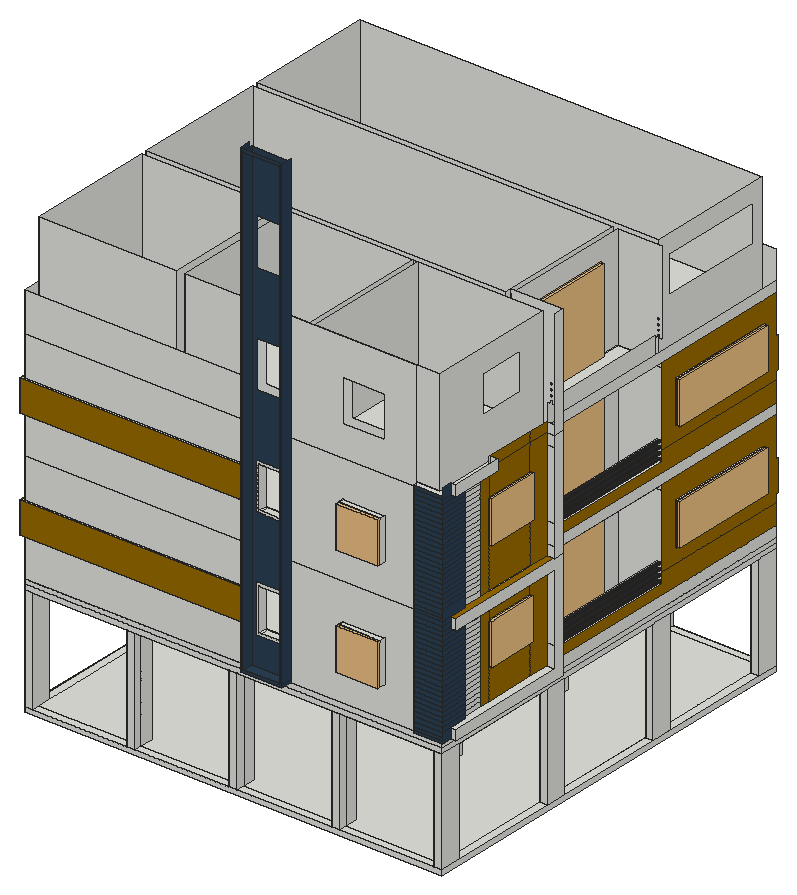
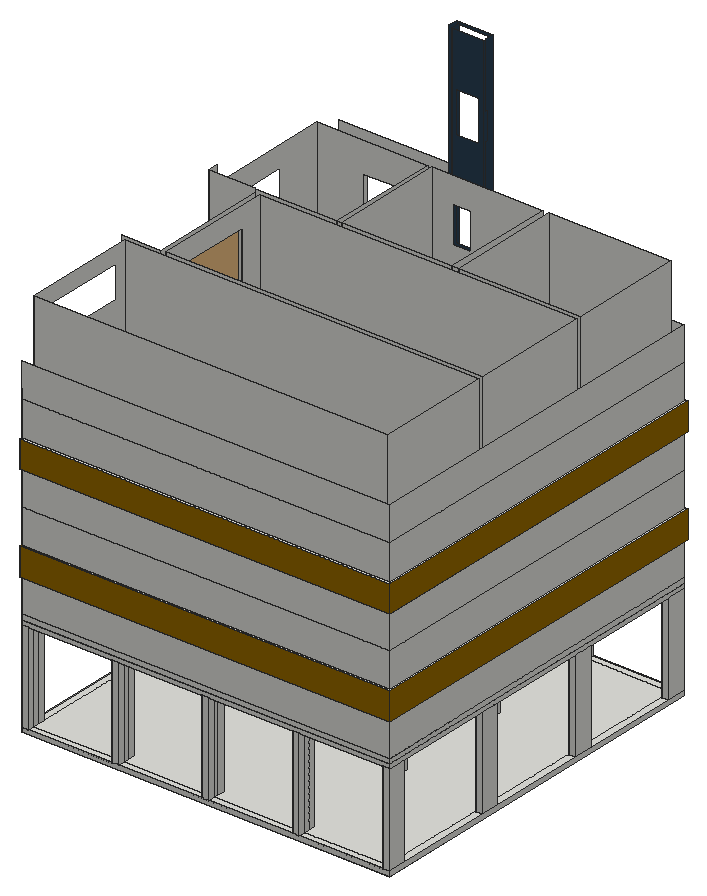
# SketchUp Ruby script. Lengths in inches.
U = 1.inch
M = Sketchup.active_model
def pt(a) = Geom::Point3d.new(a.map { |v| v * U })
def face(e, loops, mat)
  f = e.add_face(loops[0].map { |a| pt(a) })
  loops[1..].each { |l| e.add_face(l.map { |a| pt(a) }).erase! }
  f.material = f.back_material = mat if mat
  f
end
# faces: each face lists its corners as indices into pts; further lists are holes
def faces(e, pts, list, mat = nil) = list.each { |f| face(e, (f[0].is_a?(Array) ? f : [f]).map { |l| l.map { |i| pts[i] } }, mat) }
# xy, xz, yz: faces in a plane at the given z, y or x. An outline is a flat list of corners, or four numbers for a rectangle; further outlines are holes
def ring(l) = l.size == 4 ? [[l[0], l[1]], [l[2], l[1]], [l[2], l[3]], [l[0], l[3]]] : l.each_slice(2).to_a
def flat(e, list, mat, &to3) = list.each { |f| face(e, (f[0].is_a?(Array) ? f : [f]).map { |l| ring(l).map { |u, v| to3.(u, v) } }, mat) }
def xy(e, z, list, mat = nil) = flat(e, list, mat) { |x, y| [x, y, z] }
def xz(e, y, list, mat = nil) = flat(e, list, mat) { |x, z| [x, y, z] }
def yz(e, x, list, mat = nil) = flat(e, list, mat) { |y, z| [x, y, z] }
def lines(e, pts, list) = list.each { |a, b| e.add_line(pt(pts[a]), pt(pts[b])) }
# prism: a flat outline (further loops are holes) pulled along v
def prism(e, loops, v, mat = nil)
  f = face(e, loops, mat); d = Geom::Vector3d.new(v.map { |x| x * U })
  f.pushpull(f.normal.samedirection?(d) ? d.length : -d.length)
end
def box(e, o, s, mat = nil) = prism(e, [[o, [o[0] + s[0], o[1], o[2]], [o[0] + s[0], o[1] + s[1], o[2]], [o[0], o[1] + s[1], o[2]]]], [0, 0, s[2]], mat)
def at(x, y, z, deg = 0) = Geom::Transformation.translation(pt([x, y, z])) * Geom::Transformation.rotation(ORIGIN, Z_AXIS, deg.degrees)
def axes(o, x, y, z) = Geom::Transformation.new([*x, 0, *y, 0, *z, 0, *pt(o).to_a, 1])
def part(name) = M.definitions.add(name)
# library, detail: a bought-in or finely detailed component or shape, given as its bounding box
def library(name, o, s) = part(name).tap { |d| box(d.entities, o, s) }
def detail(e, o, s) = box(e.add_group.entities, o, s)
def put(e, d, t, mat = nil) = e.add_instance(d, t).tap { |i| i.material = mat if mat }
def group(e, t, mat = nil) = e.add_group.tap { |g| g.transformation = t; g.material = mat if mat }.entities
root = M.entities
M.materials.add("Carpet_04_1K").color = [43, 65, 85]
M.materials.add("D07_Ochre_Flame").color = [153, 107, 0]
M.materials.add("ThomThom - Hat1").color = [48, 46, 44]
c1 = library("mesh-163",[-551.08,-704.17,-20.03],[1929.24,1401.85,86.96])
c2 = part("Group11")
put(c2.entities,c1,at(0,0,0))
xy(root,126,[[3,12,483,492]])
xy(root,132,[[453,9,453,12,483,12,483,175,474,175,474,329,483,329,483,175,492,175,492,21.29,486,21.29,486,9],[3,12,171,21],[171,12,180,169],[180,12,324,21],[324,12,330,169],
  [330,12,483,21],[3,21,12,169],[12,21,171,169],[180,21,324,169],[330,21,474,169],
  [474,21,483,169],[3,169,3,175,426,175,426,329,3,329,3,335,483,335,483,329,432,329,432,175,483,175,483,169],[3,175,12,329],[12,175,426,329],[432,175,474,329],
  [3,335,12,492],[12,335,474,483],[474,335,483,492],[12,483,474,492]])
xy(root,132,[[261,0,309,12]],"Carpet_04_1K")
xy(root,135,[[426,202,432,302]])
xy(root,135,[[264,0,306,12]],"Carpet_04_1K")
xy(root,144,[[486,21.29,492,21.29,492,163,483,163,483,42,486,42]])
xy(root,156,[[474,175,477,329],[480,175,483,329]])
xy(root,159,[[477,175,480,329]],"ThomThom - Hat1")
xy(root,162,[[477,175,480,329]])
xy(root,165,[[477,175,480,329]],"ThomThom - Hat1")
xy(root,168,[[369,6,417,12],[477,175,480,329]])
xy(root,171,[[372,6,414,21],[273,12,276,21],[276,12,297,21]])
xy(root,171,[[477,175,480,329]],"ThomThom - Hat1")
xy(root,174,[[477,175,480,329]])
xy(root,177,[[0,9,0,495,483,495,483,492,3,492,3,12,261,12,261,9]])
xy(root,177,[[477,175,480,329]],"ThomThom - Hat1")
xy(root,183,[[474,82,483,136]])
xy(root,186,[[483,347,485,474]])
xy(root,189,[[474,350,485,471]])
xy(root,213,[[372,6,414,21],[0,9,261,9,261,12,3,12,3,492,483,492,483,495,0,495]])
xy(root,216,[[369,6,417,12]])
xy(root,219,[[273,12,297,21]])
xy(root,225,[[474,82,483,136],[426,202,432,302]])
xy(root,231,[[474,350,485,471]])
xy(root,234,[[483,347,485,474]])
xy(root,246,[[486,21.29,486,42,483,42,483,66,492,66,492,21.29],[483,66,492,163]])
xy(root,252,[[12,21,171,169],[180,21,324,169],[330,21,474,169],[171,169,180,175],[180,169,324,175],
  [324,169,330,175],[12,175,171,329],[171,175,180,329],[180,175,324,329],[324,175,330,329],
  [330,175,426,329],[171,329,180,335],[180,329,324,335],[324,329,330,335],[330,329,426,335],
  [12,335,171,483],[171,335,180,483],[180,335,324,483],[324,335,330,483],[330,335,426,483],
  [426,335,474,483]])
xy(root,258,[[12,21,171,169],[180,21,324,169],[330,21,474,169],[12,175,426,329],[432,175,474,329],
  [474,175,483,329],[12,335,474,483]])
xy(root,258,[[486,21.29,492,21.29,492,163,483,163,483,42,486,42]],"D07_Ochre_Flame")
xy(root,261,[[426,202,432,302]])
xy(root,282,[[474,175,477,329],[480,175,483,329]])
xy(root,285,[[477,175,480,329]],"ThomThom - Hat1")
xy(root,288,[[477,175,480,329]])
xy(root,291,[[477,175,480,329]],"ThomThom - Hat1")
xy(root,294,[[369,6,417,12],[477,175,480,329]])
xy(root,297,[[372,6,414,21],[273,12,276,21],[276,12,297,21]])
xy(root,297,[[477,175,480,329]],"ThomThom - Hat1")
xy(root,300,[[477,175,480,329]])
xy(root,303,[[0,9,3,492],[3,9,261,12],[0,492,483,495]])
xy(root,303,[[477,175,480,329]],"ThomThom - Hat1")
xy(root,309,[[474,82,483,136]])
xy(root,312,[[483,347,485,474]])
xy(root,315,[[474,350,485,471]])
xy(root,339,[[372,6,414,21],[0,9,3,492],[3,9,261,12],[0,492,483,495]])
xy(root,342,[[369,6,417,12]])
xy(root,345,[[273,12,297,21]])
xy(root,351,[[474,82,483,136],[426,202,432,302]])
xy(root,357,[[474,350,485,471]])
xy(root,360,[[483,347,485,474]])
xy(root,378,[[12,21,171,169],[180,21,324,169],[330,21,474,169],[171,169,180,175],[180,169,324,175],
  [324,169,330,175],[12,175,171,329],[171,175,180,329],[180,175,324,329],[324,175,330,329],
  [330,175,426,329],[171,329,180,335],[180,329,324,335],[324,329,330,335],[330,329,426,335],
  [12,335,171,483],[171,335,180,483],[180,335,324,483],[324,335,330,483],[330,335,426,483],
  [426,335,474,483]])
xy(root,384,[[180,21,324,169],[330,21,474,169],[486,21.29,486,42,483,42,483,81.29,492,81.29,492,21.29],[12,175,426,329],[432,175,474,329],
  [12,335,474,483]])
xy(root,384,[[12,21,171,169]],"D07_Ochre_Flame")
xz(root,0,[[[261,132,309,672],[264,135,306,669]]],"Carpet_04_1K")
xz(root,6,[[[369,168,417,216],[372,171,414,213]],[[369,294,417,342],[372,297,414,339]]])
xz(root,9,[[453,132,486,135.3125],[453,135.3125,486,138.625],[453,138.625,486,144],[453,144,486,149.18],[453,149.18,486,154.36],
  [453,154.36,486,159.55],[453,159.55,486,164.73],[453,164.73,486,169.91],[453,169.91,486,175.09],[453,175.09,486,180.27],
  [453,180.27,486,185.45],[453,185.45,486,190.64],[453,190.64,486,195.82],[453,195.82,486,201],[453,201,486,206.18],
  [453,206.18,486,211.36],[453,211.36,486,216.55],[453,216.55,486,221.73],[453,221.73,486,226.91],[453,226.91,486,232.09],
  [453,232.09,486,237.27],[453,237.27,486,242.45],[453,242.45,486,247.64],[453,247.64,486,252.82],[453,252.82,486,258],
  [453,258,486,261.3125],[453,261.3125,486,264.625],[453,264.625,486,270],[453,270,486,275.18],[453,275.18,486,280.36],
  [453,280.36,486,285.55],[453,285.55,486,290.73],[453,290.73,486,295.91],[453,295.91,486,301.09],[453,301.09,486,306.27],
  [453,306.27,486,311.45],[453,311.45,486,316.64],[453,316.64,486,321.82],[453,321.82,486,327],[453,327,486,332.18],
  [453,332.18,486,337.36],[453,337.36,486,342.55],[453,342.55,486,347.73],[453,347.73,486,352.91],[453,352.91,486,358.09],
  [453,358.09,486,363.27],[453,363.27,486,368.45],[453,368.45,486,373.64],[453,373.64,486,378.82],[453,378.82,486,384],
  [453,384,486,387.3125]],"Carpet_04_1K")
xz(root,9,[[0,177,261,213],[0,303,261,339]],"D07_Ochre_Flame")
xz(root,12,[[3,126,483,132],[3,132,261,177],[[309,132,453,258],[369,168,417,216]],[[270,168,300,222],[273,171,297,219]],[3,213,261,258],
  [3,258,261,303],[[309,258,453,384],[369,294,417,342]],[[270,294,300,348],[273,297,297,345]],[3,339,261,384],[3,384,261,429],
  [[309,384,453,510],[369,420,417,468]]])
xz(root,12,[[[264,135,306,669],[270,546,300,600],[270,420,300,474],[270,294,300,348],[270,168,300,222]]],"Carpet_04_1K")
xz(root,21,[[12,132,171,252],[[180,132,324,252],[273,171,297,219]],[[330,132,474,252],[372,171,414,213]],[12,258,171,378],[[180,258,324,378],[273,297,297,345]],
  [[330,258,474,378],[372,297,414,339]],[12,384,171,504],[[180,384,324,504],[273,423,297,471]],[[330,384,474,504],[372,423,414,465]]])
xz(root,21.29,[[486,132,492,144],[486,246,492,258],[486,384,492,396]])
xz(root,42,[[483,144,486,149.18],[483,149.18,486,154.36],[483,154.36,486,159.55],[483,159.55,486,164.73],[483,164.73,486,169.91],
  [483,169.91,486,175.09],[483,175.09,486,180.27],[483,180.27,486,185.45],[483,185.45,486,190.64],[483,190.64,486,195.82],
  [483,195.82,486,201],[483,201,486,206.18],[483,206.18,486,211.36],[483,211.36,486,216.55],[483,216.55,486,221.73],
  [483,221.73,486,226.91],[483,226.91,486,232.09],[483,232.09,486,237.27],[483,237.27,486,242.45],[483,242.45,486,246],
  [483,270,486,275.18],[483,275.18,486,280.36],[483,280.36,486,285.55],[483,285.55,486,290.73],[483,290.73,486,295.91],
  [483,295.91,486,301.09],[483,301.09,486,306.27],[483,306.27,486,311.45],[483,311.45,486,316.64],[483,316.64,486,321.82],
  [483,321.82,486,327],[483,327,486,332.18],[483,332.18,486,337.36],[483,337.36,486,342.55],[483,342.55,486,347.73],
  [483,347.73,486,352.91],[483,352.91,486,358.09],[483,358.09,486,363.27],[483,363.27,486,368.45],[483,368.45,486,372]])
xz(root,42,[[483,258,486,270],[483,372,486,373.64],[483,373.64,486,378.82],[483,378.82,486,383.34],[483,383.34,486,384]],"Carpet_04_1K")
xz(root,81.29,[[483,384,492,396]])
xz(root,82,[[474,183,483,225],[474,309,483,351]])
xz(root,136,[[474,183,483,225],[474,309,483,351]])
xz(root,163,[[483,144,492,168],[483,168,492,246],[483,258,492,270],[483,270,492,294],[483,294,492,372],
  [483,372,492,384],[483,384,492,396]])
xz(root,169,[[12,132,171,252],[171,132,180,252],[180,132,324,252],[324,132,330,252],[330,132,474,252],
  [12,258,171,378],[171,258,180,378],[180,258,324,378],[324,258,330,378],[330,258,474,378],
  [12,384,171,504],[171,384,180,504],[180,384,324,504],[324,384,330,504],[330,384,474,504]])
xz(root,175,[[12,132,426,252],[[432,132,432,258,492,258,492,144,483,144,483,156,480,156,480,159,477,159,477,156,474,156,474,132],[477,174,480,177],[477,162,480,165],[477,168,480,171]],[483,132,492,144],[12,258,426,378],[432,258,432,384,492,384,492,270,483,270,483,282,480,282,480,285,477,285,477,288,480,288,480,291,477,291,477,294,480,294,480,297,477,297,477,300,480,300,480,303,477,303,477,282,474,282,474,258],
  [483,258,492,270],[12,384,426,504],[[432,384,432,510,492,510,492,396,483,396,483,408,480,408,480,411,477,411,477,408,474,408,474,384],[477,426,480,429],[477,414,480,417],[477,420,480,423]],[483,384,492,396]])
xz(root,202,[[426,135,432,225],[426,261,432,351]])
xz(root,302,[[426,135,432,225],[426,261,432,351]])
xz(root,329,[[12,132,426,252],[[432,132,474,132,474,156,477,156,477,159,480,159,480,156,483,156,483,252,432,252],[477,162,480,165],[477,168,480,171],[477,174,480,177]],[432,252,483,258],[12,258,426,378],[432,258,474,258,474,282,477,282,477,303,480,303,480,300,477,300,477,297,480,297,480,294,477,294,477,291,480,291,480,288,477,288,477,285,480,285,480,282,483,282,483,378,432,378],
  [432,378,483,384],[12,384,426,504],[[432,384,474,384,474,408,477,408,477,411,480,411,480,408,483,408,483,504,432,504],[477,414,480,417],[477,420,480,423],[477,426,480,429]]])
xz(root,335,[[12,132,474,252],[12,258,474,378],[12,384,474,504]])
xz(root,347,[[483,186,485,234],[483,312,485,360]])
xz(root,350,[[474,189,485,231],[474,315,485,357]])
xz(root,471,[[474,189,485,231],[474,315,485,357]])
xz(root,474,[[483,186,485,234],[483,312,485,360]])
xz(root,483,[[12,132,474,252],[12,258,474,378],[12,384,474,504]])
xz(root,492,[[3,126,483,132],[3,132,483,177],[3,213,483,258],[3,258,483,303],[3,339,483,384],
  [3,384,483,429]])
xz(root,495,[[0,177,483,213],[0,303,483,339]],"D07_Ochre_Flame")
yz(root,0,[[9,177,495,213],[9,303,495,339]],"D07_Ochre_Flame")
yz(root,3,[[12,126,492,132],[12,132,492,177],[12,213,492,258],[12,258,492,303],[12,339,492,384],
  [12,384,492,429]])
yz(root,12,[[21,132,169,252],[175,132,329,252],[335,132,483,252],[21,258,169,378],[175,258,329,378],
  [335,258,483,378],[21,384,169,504],[175,384,329,504],[335,384,483,504]])
yz(root,171,[[21,132,169,252],[21,258,169,378],[21,384,169,504]])
yz(root,180,[[21,132,169,252],[21,258,169,378],[21,384,169,504]])
yz(root,261,[[0,132,0,672,12,672,12,588,9,588,9,552,12,552,12,465,9,465,9,429,12,429,12,339,9,339,9,303,12,303,12,213,9,213,9,177,12,177,12,132]],"Carpet_04_1K")
yz(root,264,[[0,135,12,669]],"Carpet_04_1K")
yz(root,273,[[12,171,21,219],[12,297,21,345]])
yz(root,297,[[12,171,21,210],[12,210,21,219],[12,297,21,336],[12,336,21,345]])
yz(root,306,[[0,135,12,135.3125]])
yz(root,306,[[0,135.3125,12,669]],"Carpet_04_1K")
yz(root,309,[[0,132,12,135.3125],[0,135.3125,12,672]],"Carpet_04_1K")
yz(root,324,[[21,132,169,252],[21,258,169,378],[21,384,169,504]])
yz(root,330,[[21,132,169,252],[21,258,169,378],[21,384,169,504]])
yz(root,369,[[6,168,12,216],[6,294,12,342]])
yz(root,372,[[6,171,21,213],[6,297,21,339]])
yz(root,414,[[6,171,21,213],[6,297,21,339]])
yz(root,417,[[6,168,12,216],[6,294,12,342]])
yz(root,426,[[[175,132,329,252],[202,135,302,225]],[[175,258,329,378],[202,261,302,351]],[[175,384,329,504],[202,387,302,477]]])
yz(root,432,[[175,132,199,132,199,228,305,228,305,132,329,132,329,252,175,252],[[199,132,305,228],[202,135,302,225]],[175,252,329,258],[175,258,199,258,199,354,305,354,305,258,329,258,329,378,175,378],[[199,258,305,354],[202,261,302,351]],
  [175,378,329,384],[175,384,199,384,199,480,305,480,305,384,329,384,329,504,175,504],[[199,384,305,480],[202,387,302,477]]])
yz(root,453,[[9,132,12,135.3125],[9,135.3125,12,138.625],[9,138.625,12,144],[9,144,12,149.18],[9,149.18,12,154.36],
  [9,154.36,12,159.55],[9,159.55,12,164.73],[9,164.73,12,169.91],[9,169.91,12,175.09],[9,175.09,12,180.27],
  [9,180.27,12,185.45],[9,185.45,12,190.64],[9,190.64,12,195.82],[9,195.82,12,201],[9,201,12,206.18],
  [9,206.18,12,211.36],[9,211.36,12,216.55],[9,216.55,12,221.73],[9,221.73,12,226.91],[9,226.91,12,232.09],
  [9,232.09,12,237.27],[9,237.27,12,242.45],[9,242.45,12,247.64],[9,247.64,12,252.82],[9,252.82,12,258],
  [9,258,12,261.3125],[9,261.3125,12,264.625],[9,264.625,12,270],[9,270,12,275.18],[9,275.18,12,280.36],
  [9,280.36,12,285.55],[9,285.55,12,290.73],[9,290.73,12,295.91],[9,295.91,12,301.09],[9,301.09,12,306.27],
  [9,306.27,12,311.45],[9,311.45,12,316.64],[9,316.64,12,321.82],[9,321.82,12,327],[9,327,12,332.18],
  [9,332.18,12,337.36],[9,337.36,12,342.55],[9,342.55,12,347.73],[9,347.73,12,352.91],[9,352.91,12,358.09],
  [9,358.09,12,363.27],[9,363.27,12,368.45],[9,368.45,12,373.64],[9,373.64,12,378.82],[9,378.82,12,384],
  [9,384,12,387.3125]])
yz(root,474,[[[21,132,169,252],[82,183,136,225]],[175,132,329,156],[[335,132,483,252],[350,189,471,231]],[[21,258,169,378],[82,309,136,351]],[175,258,329,282],
  [[335,258,483,378],[350,315,471,357]],[[21,384,169,504],[82,435,136,477]],[175,384,329,408],[[335,384,483,504],[350,441,471,483]]])
yz(root,477,[[175,156,329,159],[175,162,329,165],[175,168,329,171],[175,174,329,177],[175,282,329,285],
  [175,288,329,291],[175,294,329,297],[175,300,329,303]])
yz(root,480,[[175,156,329,159],[175,162,329,165],[175,168,329,171],[175,174,329,177],[175,282,329,285],
  [175,288,329,291],[175,294,329,297],[175,300,329,303]],"ThomThom - Hat1")
yz(root,483,[[12,126,492,132],[175,132,492,144],[42,144,66,149.18],[42,149.18,66,154.36],[42,154.36,66,159.55],
  [42,159.55,66,164.73],[42,164.73,66,169.91],[42,169.91,66,175.09],[42,175.09,66,180.27],[[79,180,139,228],[82,183,136,225]],
  [42,180.27,66,185.45],[42,185.45,66,190.64],[42,190.64,66,195.82],[42,195.82,66,201],[42,201,66,206.18],
  [42,206.18,66,211.36],[42,211.36,66,216.55],[42,216.55,66,221.73],[42,221.73,66,226.91],[42,226.91,66,232.09],
  [42,232.09,66,237.27],[42,237.27,66,242.45],[42,242.45,66,246],[79,246,139,258],[42,258,66,264],
  [175,258,492,270],[42,264,66,270],[42,270,66,275.18],[42,275.18,66,280.36],[42,280.36,66,285.55],
  [42,285.55,66,290.73],[42,290.73,66,295.91],[42,295.91,66,301.09],[42,301.09,66,306.27],[[79,306,139,354],[82,309,136,351]],
  [42,306.27,66,311.45],[42,311.45,66,316.64],[42,316.64,66,321.82],[42,321.82,66,327],[42,327,66,332.18],
  [42,332.18,66,337.36],[42,337.36,66,342.55],[42,342.55,66,347.73],[42,347.73,66,352.91],[42,352.91,66,358.09],
  [42,358.09,66,363.27],[42,363.27,66,368.45],[42,368.45,66,373.64],[42,373.64,66,378.82],[42,378.82,66,384],
  [79,384,81.29,396],[175,384,492,396]])
yz(root,483,[[66,144,79,246],[79,144,139,180],[139,144,163,246],[175,144,492,144,492,168,329,168,329,156,175,156],[[329,168,492,168,492,177,495,177,495,213,492,213,492,258,329,258],[347,186,474,234]],
  [79,228,139,246],[66,258,79,384],[79,258,139,306],[139,258,163,384],[175,270,492,270,492,294,329,294,329,282,175,282],
  [[329,294,492,294,492,303,495,303,495,339,492,339,492,384,329,384],[347,312,474,360]],[79,354,139,384],[81.29,384,139,396],[139,384,163,396]],"D07_Ochre_Flame")
yz(root,485,[[[347,186,474,234],[350,189,471,231]],[[347,312,474,360],[350,315,471,357]]])
yz(root,486,[[9,132,21.29,144],[9,144,42,149.18],[9,149.18,42,154.36],[9,154.36,42,159.55],[9,159.55,42,164.73],
  [9,164.73,42,169.91],[9,169.91,42,175.09],[9,175.09,42,180.27],[9,180.27,42,185.45],[9,185.45,42,190.64],
  [9,190.64,42,195.82],[9,195.82,42,201],[9,201,42,206.18],[9,206.18,42,211.36],[9,211.36,42,216.55],
  [9,216.55,42,221.73],[9,221.73,42,226.91],[9,226.91,42,232.09],[9,232.09,42,237.27],[9,237.27,42,242.45],
  [9,242.45,42,242.45,42,246,21.29,246,21.29,247.64,9,247.64],[9,247.64,21.29,252.82],[9,252.82,21.29,258],[9,258,42,270],[9,270,42,275.18],
  [9,275.18,42,280.36],[9,280.36,42,285.55],[9,285.55,42,290.73],[9,290.73,42,295.91],[9,295.91,42,301.09],
  [9,301.09,42,306.27],[9,306.27,42,311.45],[9,311.45,42,316.64],[9,316.64,42,321.82],[9,321.82,42,327],
  [9,327,42,332.18],[9,332.18,42,337.36],[9,337.36,42,342.55],[9,342.55,42,347.73],[9,347.73,42,352.91],
  [9,352.91,42,358.09],[9,358.09,42,363.27],[9,363.27,42,368.45],[9,368.45,42,373.64],[9,373.64,42,378.82],
  [9,378.82,42,384],[9,384,21.29,396]],"Carpet_04_1K")
yz(root,492,[[21.29,132,175,132,175,258,21.29,258,21.29,246,163,246,163,144,21.29,144],[163,258,175,384],[21.29,384,81.29,396],[163,384,175,510]])
p = [[324,21,378],[324,12,378],[330,21,378],[330,12,378],[474,21,378],[474,12,378],
  [474,169,378],[474,175,378],[426,483,378],[426,492,378],[330,483,378],[330,492,378],
  [324,483,378],[324,492,378],[180,483,378],[180,492,378],[474,483,378],[483,483,378],
  [474,335,378],[483,335,378],[12,335,378],[3,335,378],[324,21,252],[324,12,252],
  [330,21,252],[330,12,252],[474,21,252],[474,12,252],[474,169,252],[474,175,252],
  [426,483,252],[426,492,252],[324,483,252],[324,492,252],[180,483,252],[180,492,252],
  [474,483,252],[483,483,252],[474,335,252],[483,335,252],[12,335,252],[3,335,252],
  [477,329,159],[477,329,162],[477,175,159],[477,175,162],[477,329,165],[477,329,168],
  [477,175,165],[477,175,168],[477,329,171],[477,329,174],[477,175,171],[477,175,174]]
lines(root,p,[[0,1],[2,3],[4,5],[6,7],[8,9],[10,11],[12,13],[14,15],[16,17],[18,19],[20,21],[22,23],
  [24,25],[26,27],[28,29],[30,31],[32,33],[34,35],[36,37],[38,39],[40,41],[42,43],[44,45],[46,47],
  [48,49],[50,51],[52,53]])
g1 = group(root,at(3,12,0))
xy(g1,-6,[[-0.01,0,480,480]])
xy(g1,0,[[-0.01,0,0,24],[8.99,0,117.74,0,117.74,9,9,9,9,471,117.74,471,117.74,480,8.99,480,8.99,456.1,0,456.1,0,328.07,8.99,328.07,8.99,304.07,0,304.07,0,176.03,8.99,176.03,8.99,152.03,0,152.03,0,24,8.99,24],[126.74,0,235.49,9],[244.49,0,353.25,9],[362.25,0,471,9],
  [[9,9,117.74,9,117.74,24,126.74,24,126.74,9,235.49,9,235.49,24,244.49,24,244.49,9,353.25,9,353.25,24,362.25,24,362.25,9,471,9,471,471,362.25,471,362.25,456.1,353.25,456.1,353.25,471,244.49,471,244.49,456.1,235.49,456.1,235.49,471,126.74,471,126.74,456.1,117.74,456.1,117.74,471,9,471],[353.25,152.03,362.25,176.03],[353.25,304.07,362.25,328.07],[235.49,152.03,244.49,176.03],[235.49,304.07,244.49,328.07],[117.74,152.03,126.74,176.03],[117.74,304.07,126.74,328.07]],[-0.01,24,0,152.03],[471,24,480,152.03],[-0.01,152.03,0,176.03],[-0.01,176.03,0,304.07],
  [471,176.03,480,304.07],[-0.01,304.07,0,328.07],[-0.01,328.07,0,456.1],[471,328.07,480,456.1],[-0.01,456.1,0,480],
  [126.74,471,235.49,480],[244.49,471,353.25,480],[362.25,471,471,480],[471,480,480,480.1]])
xy(g1,120,[[0,0,8.99,24],[[8.99,0,8.99,24,0,24,0,152.03,8.99,152.03,8.99,176.03,0,176.03,0,304.07,8.99,304.07,8.99,328.07,0,328.07,0,456.1,8.99,456.1,8.99,480,117.74,480,117.74,456.1,126.74,456.1,126.74,480,235.49,480,235.49,456.1,244.49,456.1,244.49,480,353.25,480,353.25,456.1,362.25,456.1,362.25,480,471,480,471,456.1,480,456.1,480,328.07,471,328.07,471,304.07,480,304.07,480,176.03,471,176.03,471,152.03,480,152.03,480,24,471,24,471,0,362.25,0,362.25,24,353.25,24,353.25,0,244.49,0,244.49,24,235.49,24,235.49,0,126.74,0,126.74,24,117.74,24,117.74,0],[353.25,304.07,362.25,328.07],[235.49,304.07,244.49,328.07],[117.74,304.07,126.74,328.07],[353.25,152.03,362.25,176.03],[117.74,152.03,126.74,176.03],[235.49,152.03,244.49,176.03]],[117.74,0,126.74,24],[235.49,0,244.49,24],[353.25,0,362.25,24],
  [471,0,480,9],[471,9,480,24],[0,152.03,8.99,176.03],[117.74,152.03,126.74,176.03],[235.49,152.03,244.49,176.03],
  [353.25,152.03,362.25,176.03],[471,152.03,480,157],[471,157,480,161.03],[471,161.03,480,163],[471,163,480,176.03],
  [0,304.07,8.99,328.07],[117.74,304.07,126.74,328.07],[235.49,304.07,244.49,328.07],[353.25,304.07,362.25,328.07],[471,304.07,480,313.07],
  [471,313.07,480,317],[471,317,480,323],[471,323,480,328.07],[0,456.1,8.99,480],[117.74,456.1,126.74,480],
  [235.49,456.1,244.49,480],[353.25,456.1,362.25,480],[471,456.1,480,480]])
xy(g1,126,[[0,0,480,480]])
xz(g1,0,[[-0.01,-6,480,0],[0,0,8.99,120],[117.74,0,126.74,120],[235.49,0,244.49,120],[353.25,0,362.25,120],
  [471,0,480,120],[0,120,480,126]])
xz(g1,24,[[0,0,8.99,120],[117.74,0,126.74,120],[235.49,0,244.49,120],[353.25,0,362.25,120],[471,0,480,120]])
xz(g1,152.03,[[0,0,8.99,120],[117.74,0,126.74,120],[235.49,0,244.49,120],[353.25,0,362.25,120],[471,0,480,120]])
xz(g1,176.03,[[0,0,8.99,120],[117.74,0,126.74,120],[235.49,0,244.49,120],[353.25,0,362.25,120],[471,0,480,120]])
xz(g1,304.07,[[0,0,8.99,120],[117.74,0,126.74,120],[235.49,0,244.49,120],[353.25,0,362.25,120],[471,0,480,120]])
xz(g1,328.07,[[0,0,8.99,120],[117.74,0,126.74,120],[235.49,0,244.49,120],[353.25,0,362.25,120],[471,0,480,120]])
xz(g1,456.1,[[0,0,8.99,120],[117.74,0,126.74,120],[235.49,0,244.49,120],[353.25,0,362.25,120],[471,0,480,120]])
xz(g1,480,[[-0.01,-6,480,0],[0,0,8.99,120],[117.74,0,126.74,120],[235.49,0,244.49,120],[353.25,0,362.25,120],
  [471,0,480,120],[0,120,480,126]])
yz(g1,-0.01,[[0,-6,480,0]])
yz(g1,0,[[0,0,24,120],[152.03,0,176.03,120],[304.07,0,328.07,120],[456.1,0,480,120],[0,120,480,126]])
yz(g1,8.99,[[0,0,24,120],[152.03,0,176.03,120],[304.07,0,328.07,120],[456.1,0,480,120]])
yz(g1,117.74,[[0,0,9,120],[9,0,24,120],[152.03,0,157,120],[157,0,161.03,120],[161.03,0,163,120],
  [163,0,176.03,120],[304.07,0,313.07,120],[313.07,0,317,120],[317,0,323,120],[323,0,328.07,120],
  [456.1,0,465.1,120],[465.1,0,471,120],[471,0,480,120]])
yz(g1,126.74,[[0,0,9,120],[9,0,24,120],[152.03,0,176.03,120],[304.07,0,328.07,120],[456.1,0,471,120],
  [471,0,480,120]])
yz(g1,235.49,[[0,0,9,120],[9,0,24,120],[152.03,0,157,120],[157,0,161.03,120],[161.03,0,163,120],
  [163,0,176.03,120],[304.07,0,313.07,120],[313.07,0,317,120],[317,0,323,120],[323,0,328.07,120],
  [456.1,0,465.1,120],[465.1,0,471,120],[471,0,480,120]])
yz(g1,244.49,[[0,0,9,120],[9,0,24,120],[152.03,0,176.03,120],[304.07,0,328.07,120],[456.1,0,471,120],
  [471,0,480,120]])
yz(g1,353.25,[[0,0,9,120],[9,0,24,120],[152.03,0,157,120],[157,0,161.03,120],[161.03,0,163,120],
  [163,0,176.03,120],[304.07,0,313.07,120],[313.07,0,317,120],[317,0,323,120],[323,0,328.07,120],
  [456.1,0,465.1,120],[465.1,0,471,120],[471,0,480,120]])
yz(g1,362.25,[[0,0,9,120],[9,0,24,120],[152.03,0,176.03,120],[304.07,0,328.07,120],[456.1,0,471,120],
  [471,0,480,120]])
yz(g1,471,[[0,0,9,120],[9,0,24,120],[152.03,0,157,120],[157,0,161.03,120],[161.03,0,163,120],
  [163,0,176.03,120],[304.07,0,313.07,120],[313.07,0,317,120],[317,0,323,120],[323,0,328.07,120],
  [456.1,0,465.1,120],[465.1,0,471,120],[471,0,480,120]])
yz(g1,480,[[0,-6,480,0],[0,0,24,120],[152.03,0,176.03,120],[304.07,0,328.07,120],[456.1,0,480,120],
  [0,120,480,126]])
put(root,c2,axes([432.79,229.16,181.03],[0,0.05472,0],[0,0,0.06732],[0.03937,0,0]))
put(root,c2,axes([382.71,5.21,192.1],[0.02488,0,0],[0,0,0.03425],[0,-0.03937,0]))
put(root,c2,axes([483.79,96.09,204.38],[0,0.03102,0],[0,0,0.03386],[0.03937,0,0]))
put(root,c2,axes([485.79,383.28,210.38],[0,0.06583,0],[0,0,0.03386],[0.03937,0,0]))
put(root,c2,axes([432.79,229.16,306.22],[0,0.05472,0],[0,0,0.06848],[0.03937,0,0]))
put(root,c2,axes([382.67,5.21,318.1],[0.0248,0,0],[0,0,0.03425],[0,-0.03937,0]))
put(root,c2,axes([483.79,96.36,330.1],[0,0.0315,0],[0,0,0.03425],[0.03937,0,0]))
put(root,c2,axes([485.79,383.45,336.1],[0,0.06614,0],[0,0,0.03425],[0.03937,0,0]))
put(root,c2,axes([432.79,229.16,432.22],[0,0.05472,0],[0,0,0.06848],[0.03937,0,0]))
